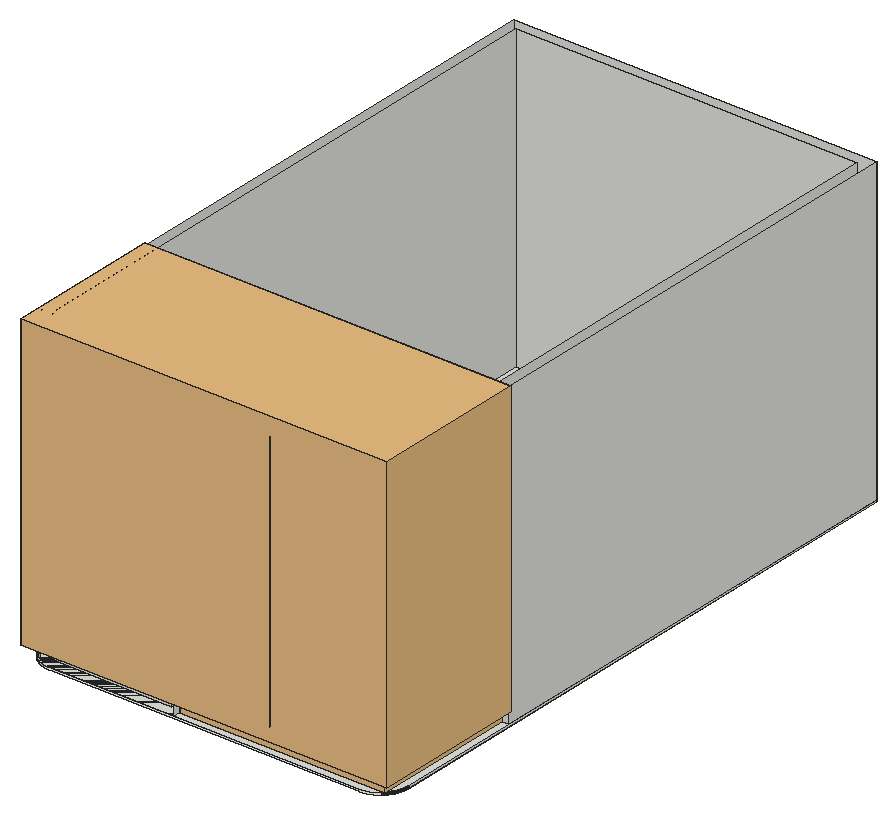
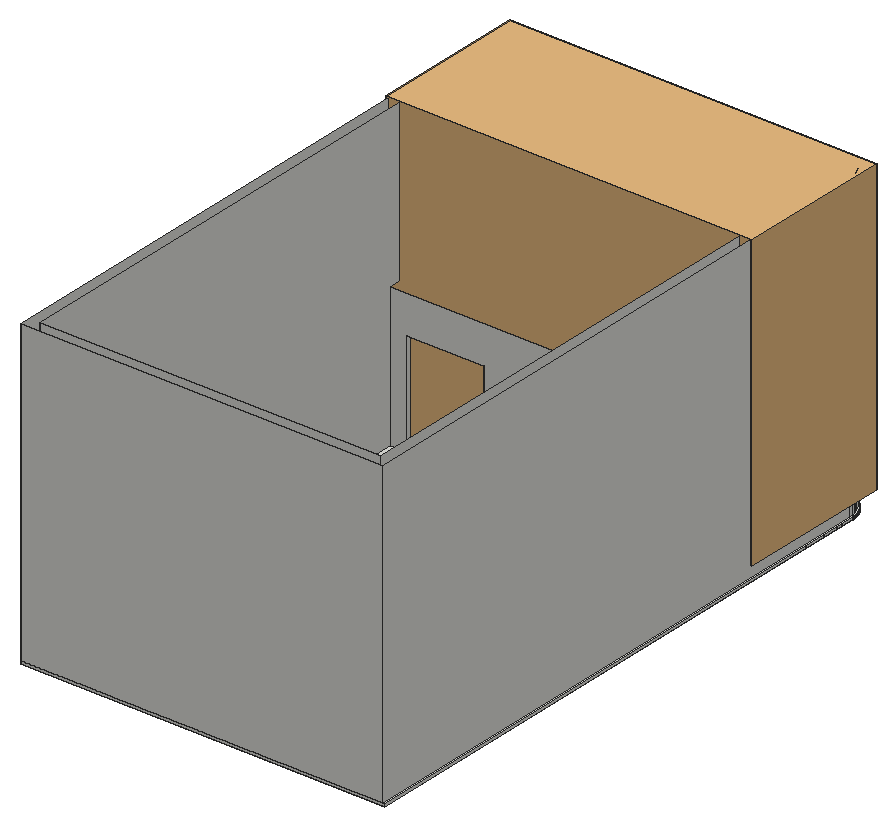
# SketchUp Ruby script. Lengths in inches.
U = 1.inch
M = Sketchup.active_model
def pt(a) = Geom::Point3d.new(a.map { |v| v * U })
def face(e, loops, mat)
  f = e.add_face(loops[0].map { |a| pt(a) })
  loops[1..].each { |l| e.add_face(l.map { |a| pt(a) }).erase! }
  f.material = f.back_material = mat if mat
  f
end
# faces: each face lists its corners as indices into pts; further lists are holes
def faces(e, pts, list, mat = nil) = list.each { |f| face(e, (f[0].is_a?(Array) ? f : [f]).map { |l| l.map { |i| pts[i] } }, mat) }
# xy, xz, yz: faces in a plane at the given z, y or x. An outline is a flat list of corners, or four numbers for a rectangle; further outlines are holes
def ring(l) = l.size == 4 ? [[l[0], l[1]], [l[2], l[1]], [l[2], l[3]], [l[0], l[3]]] : l.each_slice(2).to_a
def flat(e, list, mat, &to3) = list.each { |f| face(e, (f[0].is_a?(Array) ? f : [f]).map { |l| ring(l).map { |u, v| to3.(u, v) } }, mat) }
def xy(e, z, list, mat = nil) = flat(e, list, mat) { |x, y| [x, y, z] }
def xz(e, y, list, mat = nil) = flat(e, list, mat) { |x, z| [x, y, z] }
def yz(e, x, list, mat = nil) = flat(e, list, mat) { |y, z| [x, y, z] }
def lines(e, pts, list) = list.each { |a, b| e.add_line(pt(pts[a]), pt(pts[b])) }
# prism: a flat outline (further loops are holes) pulled along v
def prism(e, loops, v, mat = nil)
  f = face(e, loops, mat); d = Geom::Vector3d.new(v.map { |x| x * U })
  f.pushpull(f.normal.samedirection?(d) ? d.length : -d.length)
end
def box(e, o, s, mat = nil) = prism(e, [[o, [o[0] + s[0], o[1], o[2]], [o[0] + s[0], o[1] + s[1], o[2]], [o[0], o[1] + s[1], o[2]]]], [0, 0, s[2]], mat)
def at(x, y, z, deg = 0) = Geom::Transformation.translation(pt([x, y, z])) * Geom::Transformation.rotation(ORIGIN, Z_AXIS, deg.degrees)
def axes(o, x, y, z) = Geom::Transformation.new([*x, 0, *y, 0, *z, 0, *pt(o).to_a, 1])
def part(name) = M.definitions.add(name)
# library, detail: a bought-in or finely detailed component or shape, given as its bounding box
def library(name, o, s) = part(name).tap { |d| box(d.entities, o, s) }
def detail(e, o, s) = box(e.add_group.entities, o, s)
def put(e, d, t, mat = nil) = e.add_instance(d, t).tap { |i| i.material = mat if mat }
def group(e, t, mat = nil) = e.add_group.tap { |g| g.transformation = t; g.material = mat if mat }.entities
root = M.entities
c1 = library("Group\#6",[0,0,0],[316.03,134.01,252])
c2 = library("Group\#7",[0,-2,0],[117,2,225.22])
c3 = library("Group\#11",[0,0,0],[177.45,126,38])
c4 = library("SLIDING+GLASS+DOOR",[0,-0.75,0],[72,5.75,80])
xy(root,126,[[17.86,155,17.73,155.01,17.59,155.01,17.45,155.02,17.3125,155.03,17.18,155.05,16.9,155.09,16.77,155.11,16.63,155.13,16.37,155.19,16.23,155.23,16.1,155.26,15.84,155.34,15.71,155.39,15.58,155.43,15.32,155.53,15.19,155.59,15.07,155.64,14.95,155.7,14.82,155.76,14.7,155.83,14.58,155.89,14.34,156.03,14.23,156.1,14.11,156.18,13.67,156.5,13.45,156.68,13.15,156.95,12.95,157.15,12.68,157.45,12.5,157.67,12.18,158.11,12.1,158.23,12.03,158.34,11.89,158.58,11.83,158.7,11.76,158.82,11.7,158.95,11.64,159.07,11.59,159.19,11.53,159.32,11.43,159.58,11.39,159.71,11.34,159.84,11.26,160.1,11.23,160.23,11.19,160.37,11.13,160.63,11.11,160.77,11.09,160.9,11.05,161.18,11.03,161.3125,11.02,161.45,11.01,161.59,11.01,161.73,11,161.86,11,190,156.05,190,156.05,334,303.45,334,303.45,162,303.39,161.09,303.21,160.1875,302.92,159.32,302.52,158.5,302.01,157.74,301.4,157.05,300.71,156.45,299.95,155.9375,299.13,155.53,298.27,155.24,297.37,155.06,296.45,155]])
xy(root,130,[[[23.87,144,23.56,144.01,22.92,144.03,22.61,144.05,22.29,144.07,21.98,144.1,21.66,144.13,21.35,144.17,21.03,144.21,20.72,144.25,20.4,144.3,19.78,144.4,19.16,144.52,18.54,144.66,18.23,144.74,17.93,144.82,17.62,144.9,17.02,145.08,16.71,145.17,16.41,145.27,16.11,145.375,15.82,145.48,15.52,145.59,15.23,145.71,14.93,145.83,14.35,146.07,14.0625,146.2,13.78,146.34,13.49,146.48,12.93,146.76,12.37,147.06,12.09,147.22,11.82,147.375,11.55,147.54,11.28,147.7,11.01,147.87,10.75,148.04,9.97,148.58,9.72,148.77,9.46,148.96,9.21,149.15,8.97,149.35,8.72,149.55,8.48,149.75,8.24,149.96,8,150.16,7.54,150.59,7.08,151.03,6.86,151.25,6.64,151.48,6.43,151.71,6.21,151.94,6,152.18,5.8,152.41,5.59,152.65,5.39,152.9,5.19,153.14,4.62,153.89,4.44,154.15,4.25,154.41,4.08,154.67,3.9,154.93,3.73,155.19,3.5625,155.46,3.4,155.73,3.08,156.27,2.78,156.83,2.64,157.1,2.49,157.39,2.36,157.67,2.22,157.95,1.96,158.53,1.72,159.11,1.5,159.69,1.28,160.29,1.18,160.58,1,161.18,0.91,161.49,0.82,161.79,0.74,162.09,0.67,162.4,0.6,162.7,0.46,163.32,0.41,163.625,0.35,163.9375,0.3,164.25,0.25,164.56,0.13,165.49,0.1,165.8,0.07,166.12,0.03,166.74,0.02,167.06,0.01,167.37,0,167.6875,0,672,314.45,672,314.45,167.37,314.43,167.06,314.42,166.74,314.38,166.12,314.35,165.8,314.29,165.18,314.25,164.87,314.2,164.56,314.16,164.25,314.1,163.9375,314.05,163.625,313.99,163.32,313.92,163.01,313.86,162.7,313.79,162.4,313.71,162.09,313.55,161.49,313.46,161.18,313.37,160.88,313.27,160.58,313.17,160.29,313.07,159.99,312.96,159.69,312.85,159.4,312.49,158.53,312.23,157.95,312.1,157.67,311.96,157.39,311.82,157.1,311.67,156.83,311.37,156.27,310.89,155.46,310.72,155.19,310.55,154.93,310.2,154.41,310.02,154.15,309.83,153.89,309.65,153.64,309.45,153.39,309.26,153.14,309.0625,152.9,308.86,152.65,308.66,152.41,308.45,152.18,308.24,151.94,308.03,151.71,307.8125,151.48,307.59,151.25,307.37,151.03,307.14,150.81,306.92,150.59,306.68,150.375,306.45,150.16,306.21,149.96,305.97,149.75,305.49,149.35,305.24,149.15,304.74,148.77,304.48,148.58,304.23,148.4,303.97,148.22,303.7,148.04,303.4375,147.87,303.17,147.7,302.9,147.54,302.63,147.375,302.36,147.22,302.08,147.06,301.81,146.91,301.53,146.76,301.25,146.62,300.96,146.48,300.68,146.34,300.39,146.2,300.1,146.07,299.8125,145.95,299.52,145.83,299.23,145.71,298.93,145.59,298.64,145.48,298.04,145.27,297.74,145.17,297.4375,145.08,297.13,144.99,296.83,144.9,296.53,144.82,295.91,144.66,295.29,144.52,294.67,144.4,293.74,144.25,293.42,144.21,293.11,144.17,292.79,144.13,292.48,144.1,292.16,144.07,291.85,144.05,291.53,144.03,291.21,144.02,290.9,144.01,290.58,144],[23.9,146,290.55,146,290.85,146.01,291.43,146.03,291.71,146.05,292.29,146.09,292.87,146.15,293.16,146.1875,293.45,146.23,293.73,146.27,294.31,146.37,294.59,146.42,295.16,146.54,296,146.75,296.28,146.83,296.5625,146.91,296.84,146.99,297.12,147.08,297.39,147.17,297.67,147.26,297.9375,147.36,298.21,147.46,298.48,147.57,298.75,147.67,299.02,147.79,299.28,147.9,299.55,148.02,299.81,148.14,300.59,148.53,300.84,148.67,301.1,148.81,301.6,149.09,302.1,149.39,302.82,149.87,303.0625,150.03,303.3,150.2,303.53,150.37,303.76,150.55,303.99,150.72,304.22,150.9,304.44,151.09,304.66,151.27,305.32,151.84,305.74,152.24,306.15,152.65,306.55,153.07,306.74,153.28,306.94,153.49,307.125,153.71,307.5,154.15,307.86,154.61,308.37,155.3,308.54,155.54,309.02,156.26,309.17,156.51,309.32,156.75,309.47,157,309.75,157.5,309.89,157.76,310.02,158.01,310.28,158.53,310.52,159.05,310.64,159.32,310.75,159.58,310.86,159.85,310.96,160.12,311.07,160.39,311.17,160.66,311.35,161.2,311.44,161.48,311.52,161.75,311.61,162.03,311.68,162.31,311.76,162.58,311.83,162.86,311.89,163.14,311.95,163.43,312.07,163.99,312.12,164.27,312.16,164.56,312.21,164.84,312.25,165.13,312.28,165.41,312.32,165.7,312.34,165.99,312.37,166.27,312.39,166.5625,312.41,166.85,312.42,167.14,312.43,167.42,312.4375,167.71,312.4375,670,2.02,670,2.02,167.42,2.03,167.14,2.05,166.85,2.0625,166.5625,2.08,166.27,2.11,165.99,2.17,165.41,2.21,165.13,2.25,164.84,2.29,164.56,2.34,164.27,2.44,163.71,2.5,163.43,2.5625,163.14,2.63,162.86,2.7,162.58,2.77,162.31,2.93,161.75,3.01,161.48,3.1,161.2,3.19,160.93,3.59,159.85,3.7,159.58,3.82,159.32,3.93,159.05,4.05,158.79,4.18,158.53,4.3,158.27,4.43,158.01,4.57,157.76,4.7,157.5,4.84,157.25,4.99,157,5.13,156.75,5.28,156.51,5.4375,156.26,5.59,156.02,5.75,155.78,5.92,155.54,6.08,155.3,6.42,154.84,6.96,154.15,7.14,153.93,7.52,153.49,7.71,153.28,8.51,152.44,9.14,151.84,9.35,151.65,9.79,151.27,10.01,151.09,10.23,150.9,10.46,150.72,10.69,150.55,10.92,150.37,11.16,150.2,11.39,150.03,12.11,149.55,12.36,149.39,12.6,149.24,12.85,149.09,13.35,148.81,13.61,148.67,13.86,148.53,14.64,148.14,14.91,148.02,15.17,147.9,15.4375,147.79,15.7,147.67,15.97,147.57,16.24,147.46,16.51,147.36,16.79,147.26,17.0625,147.17,17.34,147.08,17.61,146.99,18.45,146.75,19.01,146.61,19.3,146.54,19.86,146.42,20.15,146.37,20.43,146.32,20.72,146.27,21.01,146.23,21.29,146.1875,21.58,146.15,22.16,146.09,23.03,146.03]]])
xy(root,132,[[23.87,144,290.58,144,290.9,144.01,291.21,144.02,291.53,144.03,291.85,144.05,292.16,144.07,292.48,144.1,292.79,144.13,293.11,144.17,293.42,144.21,293.74,144.25,294.67,144.4,295.29,144.52,295.91,144.66,296.53,144.82,296.83,144.9,297.13,144.99,297.4375,145.08,297.74,145.17,298.04,145.27,298.64,145.48,298.93,145.59,299.23,145.71,299.52,145.83,299.8125,145.95,300.1,146.07,300.39,146.2,300.68,146.34,300.96,146.48,301.25,146.62,301.53,146.76,301.81,146.91,302.08,147.06,302.36,147.22,302.63,147.375,302.9,147.54,303.17,147.7,303.4375,147.87,303.7,148.04,303.97,148.22,304.23,148.4,304.48,148.58,304.74,148.77,305.24,149.15,305.49,149.35,305.97,149.75,306.21,149.96,306.45,150.16,306.68,150.375,306.92,150.59,307.14,150.81,307.37,151.03,307.59,151.25,307.8125,151.48,308.03,151.71,308.24,151.94,308.45,152.18,308.66,152.41,308.86,152.65,309.0625,152.9,309.26,153.14,309.45,153.39,309.65,153.64,309.83,153.89,310.02,154.15,310.2,154.41,310.55,154.93,310.72,155.19,310.89,155.46,311.37,156.27,311.67,156.83,311.82,157.1,311.96,157.39,312.1,157.67,312.23,157.95,312.49,158.53,312.85,159.4,312.96,159.69,313.07,159.99,313.17,160.29,313.27,160.58,313.37,160.88,313.46,161.18,313.55,161.49,313.71,162.09,313.79,162.4,313.86,162.7,313.92,163.01,313.99,163.32,314.05,163.625,314.1,163.9375,314.16,164.25,314.2,164.56,314.25,164.87,314.29,165.18,314.35,165.8,314.38,166.12,314.42,166.74,314.43,167.06,314.45,167.37,314.45,672,0,672,0,167.6875,0.01,167.37,0.02,167.06,0.03,166.74,0.07,166.12,0.1,165.8,0.13,165.49,0.25,164.56,0.3,164.25,0.35,163.9375,0.41,163.625,0.46,163.32,0.6,162.7,0.67,162.4,0.74,162.09,0.82,161.79,0.91,161.49,1,161.18,1.18,160.58,1.28,160.29,1.5,159.69,1.72,159.11,1.96,158.53,2.22,157.95,2.36,157.67,2.49,157.39,2.64,157.1,2.78,156.83,3.08,156.27,3.4,155.73,3.5625,155.46,3.73,155.19,3.9,154.93,4.08,154.67,4.25,154.41,4.44,154.15,4.62,153.89,5.19,153.14,5.39,152.9,5.59,152.65,5.8,152.41,6,152.18,6.21,151.94,6.43,151.71,6.64,151.48,6.86,151.25,7.08,151.03,7.54,150.59,8,150.16,8.24,149.96,8.48,149.75,8.72,149.55,8.97,149.35,9.21,149.15,9.46,148.96,9.72,148.77,9.97,148.58,10.75,148.04,11.01,147.87,11.28,147.7,11.55,147.54,11.82,147.375,12.09,147.22,12.37,147.06,12.93,146.76,13.49,146.48,13.78,146.34,14.0625,146.2,14.35,146.07,14.93,145.83,15.23,145.71,15.52,145.59,15.82,145.48,16.11,145.375,16.41,145.27,16.71,145.17,17.02,145.08,17.62,144.9,17.93,144.82,18.23,144.74,18.54,144.66,19.16,144.52,19.78,144.4,20.4,144.3,20.72,144.25,21.03,144.21,21.35,144.17,21.66,144.13,21.98,144.1,22.29,144.07,22.61,144.05,22.92,144.03,23.56,144.01],[26,144,22.87,144.21,19.79,144.82,16.82,145.83,14,147.22,11.39,148.96,9.03,151.03,6.96,153.39,5.22,156,3.83,158.82,2.82,161.79,2.21,164.87,2,168,2,672,314.45,672,314.45,276,290.45,276,290.45,285,305,285,305,663,11,663,11,168,11.13,166.04,11.51,164.12,12.14,162.26,13.01,160.5,14.1,158.87,15.39,157.4,16.87,156.1,18.5,155.01,20.26,154.14,22.12,153.51,24.04,153.13,26,153,122,153,122,285,131,285,131,144],[131,276,224.45,285]])
xz(root,153,[[26,132,26,392.81,290.45,392.81,290.45,254.81,122,254.81,122,132]])
xz(root,276,[[131,132,224.45,132,224.45,222,290.45,222,290.45,132,314.45,132,314.45,251,131,251]])
xz(root,285,[[122,132,122,254.81,305,254.81,305,132,290.45,132,290.45,222,224.45,222,224.45,132]])
xz(root,663,[[11,132,305,392.81]])
xz(root,672,[[0,130,314.45,132],[2,132,314.45,392.81]])
yz(root,0,[[167.6875,130,168,132],[168,130,672,132]])
yz(root,2,[[168,132,672,392.81]])
yz(root,11,[[168,132,663,392.81]])
yz(root,122,[[153,132,285,254.81]])
yz(root,131,[[144,132,276,132,276,251,146,251,146,144.28,144,144.28]])
yz(root,224.45,[[276,132,285,222]])
yz(root,290.45,[[276,132,285,222]])
yz(root,305,[[285,132,285,254.81,164.34,254.81,164.34,392.81,663,392.81,663,132]])
yz(root,314.45,[[167.37,130,167.6875,132],[167.6875,130,168,132],[168,130,672,132],[276,132,672,132,672,392.81,168,392.81,168,251,276,251]])
p = [[8.48,149.75,130],[8.72,149.55,130],[8.72,149.55,132],[8.48,149.75,132],[305.73,149.55,130],[305.97,149.75,130],
  [305.97,149.75,132],[305.73,149.55,132],[8.24,149.96,130],[8.24,149.96,132],[306.21,149.96,130],[306.21,149.96,132],
  [8,150.16,130],[8,150.16,132],[306.45,150.16,130],[306.45,150.16,132],[7.77,150.375,130],[7.77,150.375,132],
  [306.68,150.375,130],[306.68,150.375,132],[7.54,150.59,130],[7.54,150.59,132],[306.92,150.59,130],[306.92,150.59,132],
  [7.31,150.81,130],[7.31,150.81,132],[307.14,150.81,130],[307.14,150.81,132],[7.08,151.03,130],[7.08,151.03,132],
  [307.37,151.03,130],[307.37,151.03,132],[6.86,151.25,130],[6.86,151.25,132],[307.59,151.25,130],[307.59,151.25,132],
  [6.64,151.48,130],[6.64,151.48,132],[307.8125,151.48,130],[307.8125,151.48,132],[6.43,151.71,130],[6.43,151.71,132],
  [308.03,151.71,130],[308.03,151.71,132],[6.21,151.94,130],[6.21,151.94,132],[308.24,151.94,130],[308.24,151.94,132],
  [6,152.18,130],[6,152.18,132],[308.45,152.18,130],[308.45,152.18,132],[5.8,152.41,130],[5.8,152.41,132],
  [308.66,152.41,130],[308.66,152.41,132],[5.59,152.65,130],[5.59,152.65,132],[308.86,152.65,130],[308.86,152.65,132],
  [5.39,152.9,130],[5.39,152.9,132],[309.0625,152.9,130],[309.0625,152.9,132],[5.19,153.14,130],[5.19,153.14,132],
  [309.26,153.14,130],[309.26,153.14,132],[5,153.39,130],[5,153.39,132],[309.45,153.39,130],[309.45,153.39,132],
  [4.81,153.64,130],[4.81,153.64,132],[309.65,153.64,130],[309.65,153.64,132],[4.62,153.89,130],[4.62,153.89,132],
  [309.83,153.89,130],[309.83,153.89,132],[4.44,154.15,130],[4.44,154.15,132],[310.02,154.15,130],[310.02,154.15,132],
  [4.25,154.41,130],[4.25,154.41,132],[310.2,154.41,130],[310.2,154.41,132],[4.08,154.67,130],[4.08,154.67,132],
  [310.375,154.67,130],[310.375,154.67,132],[3.9,154.93,130],[3.9,154.93,132],[310.55,154.93,130],[310.55,154.93,132],
  [3.73,155.19,130],[3.73,155.19,132],[310.72,155.19,130],[310.72,155.19,132],[3.5625,155.46,130],[3.5625,155.46,132],
  [310.89,155.46,130],[310.89,155.46,132],[3.4,155.73,130],[3.4,155.73,132],[311.05,155.73,130],[311.05,155.73,132],
  [3.24,156,130],[3.24,156,132],[311.21,156,130],[311.21,156,132],[3.08,156.27,130],[3.08,156.27,132],
  [311.37,156.27,130],[311.37,156.27,132],[2.93,156.55,130],[2.93,156.55,132],[311.52,156.55,130],[311.52,156.55,132],
  [2.78,156.83,130],[2.78,156.83,132],[311.67,156.83,130],[311.67,156.83,132],[2.64,157.1,130],[2.64,157.1,132],
  [311.82,157.1,130],[311.82,157.1,132],[2.49,157.39,130],[2.49,157.39,132],[311.96,157.39,130],[311.96,157.39,132],
  [2.36,157.67,130],[2.36,157.67,132],[312.1,157.67,130],[312.1,157.67,132],[2.22,157.95,130],[2.22,157.95,132],
  [312.23,157.95,130],[312.23,157.95,132],[2.09,158.24,130],[2.09,158.24,132],[312.36,158.24,130],[312.36,158.24,132],
  [1.96,158.53,130],[1.96,158.53,132],[312.49,158.53,130],[312.49,158.53,132],[1.84,158.82,130],[1.84,158.82,132],
  [312.61,158.82,130],[312.61,158.82,132],[1.72,159.11,130],[1.72,159.11,132],[312.73,159.11,130],[312.73,159.11,132],
  [1.61,159.4,130],[1.61,159.4,132],[312.85,159.4,130],[312.85,159.4,132],[1.5,159.69,130],[1.5,159.69,132],
  [312.96,159.69,130],[312.96,159.69,132],[1.39,159.99,130],[1.39,159.99,132],[313.07,159.99,130],[313.07,159.99,132],
  [1.28,160.29,130],[1.28,160.29,132],[313.17,160.29,130],[313.17,160.29,132],[1.18,160.58,130],[1.18,160.58,132],
  [313.27,160.58,130],[313.27,160.58,132],[1.09,160.88,130],[1.09,160.88,132],[313.37,160.88,130],[313.37,160.88,132],
  [1,161.18,130],[1,161.18,132],[313.46,161.18,130],[313.46,161.18,132],[0.91,161.49,130],[0.91,161.49,132],
  [313.55,161.49,130],[313.55,161.49,132],[0.82,161.79,130],[0.82,161.79,132],[313.63,161.79,130],[313.63,161.79,132],
  [0.74,162.09,130],[0.74,162.09,132],[313.71,162.09,130],[313.71,162.09,132],[0.67,162.4,130],[0.67,162.4,132],
  [313.79,162.4,130],[313.79,162.4,132],[0.6,162.7,130],[0.6,162.7,132],[313.86,162.7,130],[313.86,162.7,132],
  [0.53,163.01,130],[0.53,163.01,132],[313.92,163.01,130],[313.92,163.01,132],[0.46,163.32,130],[0.46,163.32,132],
  [313.99,163.32,130],[313.99,163.32,132],[0.41,163.625,130],[0.41,163.625,132],[314.05,163.625,130],[314.05,163.625,132],
  [0.35,163.9375,130],[0.35,163.9375,132],[314.1,163.9375,130],[314.1,163.9375,132],[0.3,164.25,130],[0.3,164.25,132],
  [314.16,164.25,130],[314.16,164.25,132],[0.25,164.56,130],[0.25,164.56,132],[314.2,164.56,130],[314.2,164.56,132],
  [0.21,164.87,130],[0.21,164.87,132],[314.25,164.87,130],[314.25,164.87,132],[0.17,165.18,130],[0.17,165.18,132],
  [314.29,165.18,130],[314.29,165.18,132],[0.13,165.49,130],[0.13,165.49,132],[314.32,165.49,130],[314.32,165.49,132],
  [0.1,165.8,130],[0.1,165.8,132],[314.35,165.8,130],[314.35,165.8,132],[0.07,166.12,130],[0.07,166.12,132],
  [314.38,166.12,130],[314.38,166.12,132],[0.05,166.43,130],[0.05,166.43,132],[314.4,166.43,130],[314.4,166.43,132],
  [0.03,166.74,130],[0.03,166.74,132],[314.42,166.74,130],[314.42,166.74,132],[0.02,167.06,130],[0.02,167.06,132],
  [314.43,167.06,130],[314.43,167.06,132],[0.01,167.37,130],[0.01,167.37,132],[314.45,167.37,130],[314.45,167.37,132],
  [0,167.6875,130],[0,167.6875,132],[9.03,151.03,132],[11.39,148.96,132],[11.39,148.96,392.81],[9.03,151.03,392.81],
  [6.96,153.39,132],[6.96,153.39,392.81],[26,153,132],[24.04,153.13,132],[24.04,153.13,392.81],[26,153,392.81],
  [22.12,153.51,132],[22.12,153.51,392.81],[5.22,156,132],[5.22,156,392.81],[20.26,154.14,132],[20.26,154.14,392.81],
  [18.5,155.01,132],[18.5,155.01,392.81],[16.87,156.1,132],[16.87,156.1,392.81],[3.83,158.82,132],[3.83,158.82,392.81],
  [15.39,157.4,132],[15.39,157.4,392.81],[14.1,158.87,132],[14.1,158.87,392.81],[2.82,161.79,132],[2.82,161.79,392.81],
  [13.01,160.5,132],[13.01,160.5,392.81],[12.14,162.26,132],[12.14,162.26,392.81],[2.21,164.87,132],[2.21,164.87,392.81],
  [11.51,164.12,132],[11.51,164.12,392.81],[11.13,166.04,132],[11.13,166.04,392.81],[2,168,132],[2,168,392.81],
  [11,168,132],[11,168,392.81],[306.95,451.62,132],[314.45,451.62,132]]
faces(root,p,[[0,1,2,3],[4,5,6,7],[8,0,3,9],[5,10,11,6],[12,8,9,13],[10,14,15,11],[16,12,13,17],[14,18,19,15],
  [20,16,17,21],[18,22,23,19],[24,20,21,25],[22,26,27,23],[28,24,25,29],[26,30,31,27],[32,28,29,33],[30,34,35,31],
  [36,32,33,37],[34,38,39,35],[40,36,37,41],[38,42,43,39],[44,40,41,45],[42,46,47,43],[48,44,45,49],[46,50,51,47],
  [52,48,49,53],[50,54,55,51],[56,52,53,57],[54,58,59,55],[60,56,57,61],[58,62,63,59],[64,60,61,65],[62,66,67,63],
  [68,64,65,69],[66,70,71,67],[72,68,69,73],[70,74,75,71],[76,72,73,77],[74,78,79,75],[80,76,77,81],[78,82,83,79],
  [84,80,81,85],[82,86,87,83],[88,84,85,89],[86,90,91,87],[92,88,89,93],[90,94,95,91],[96,92,93,97],[94,98,99,95],
  [100,96,97,101],[98,102,103,99],[104,100,101,105],[102,106,107,103],[108,104,105,109],[106,110,111,107],[112,108,109,113],[110,114,115,111],
  [116,112,113,117],[114,118,119,115],[120,116,117,121],[118,122,123,119],[124,120,121,125],[122,126,127,123],[128,124,125,129],[126,130,131,127],
  [132,128,129,133],[130,134,135,131],[136,132,133,137],[134,138,139,135],[140,136,137,141],[138,142,143,139],[144,140,141,145],[142,146,147,143],
  [148,144,145,149],[146,150,151,147],[152,148,149,153],[150,154,155,151],[156,152,153,157],[154,158,159,155],[160,156,157,161],[158,162,163,159],
  [164,160,161,165],[162,166,167,163],[168,164,165,169],[166,170,171,167],[172,168,169,173],[170,174,175,171],[176,172,173,177],[174,178,179,175],
  [180,176,177,181],[178,182,183,179],[184,180,181,185],[182,186,187,183],[188,184,185,189],[186,190,191,187],[192,188,189,193],[190,194,195,191],
  [196,192,193,197],[194,198,199,195],[200,196,197,201],[198,202,203,199],[204,200,201,205],[202,206,207,203],[208,204,205,209],[206,210,211,207],
  [212,208,209,213],[210,214,215,211],[216,212,213,217],[214,218,219,215],[220,216,217,221],[218,222,223,219],[224,220,221,225],[222,226,227,223],
  [228,224,225,229],[226,230,231,227],[232,228,229,233],[230,234,235,231],[236,232,233,237],[234,238,239,235],[240,236,237,241],[238,242,243,239],
  [244,240,241,245],[242,246,247,243],[248,244,245,249],[246,250,251,247],[252,248,249,253],[250,254,255,251],[256,252,253,257],[254,258,259,255],
  [260,256,257,261],[258,262,263,259],[264,260,261,265],[266,267,268,269],[270,266,269,271],[272,273,274,275],[273,276,277,274],[278,270,271,279],
  [276,280,281,277],[280,282,283,281],[282,284,285,283],[286,278,279,287],[284,288,289,285],[288,290,291,289],[292,286,287,293],[290,294,295,291],
  [294,296,297,295],[298,292,293,299],[296,300,301,297],[300,302,303,301],[304,298,299,305],[302,306,307,303]])
lines(root,p,[[308,309]])
put(root,c1,at(0,142,142))
g1 = group(root,at(1,143.5,154))
detail(g1,[0,0,0],[95.27,24,228])
put(g1,c2,axes([95.27,1,0],[1.01505,0,0],[0,1,0],[0,0,1]))
put(g1,c3,at(130,6.5,-22))
put(root,c4,axes([224.45,277,132],[0.91667,0,0],[0,1,0],[0,0,1.125]))
